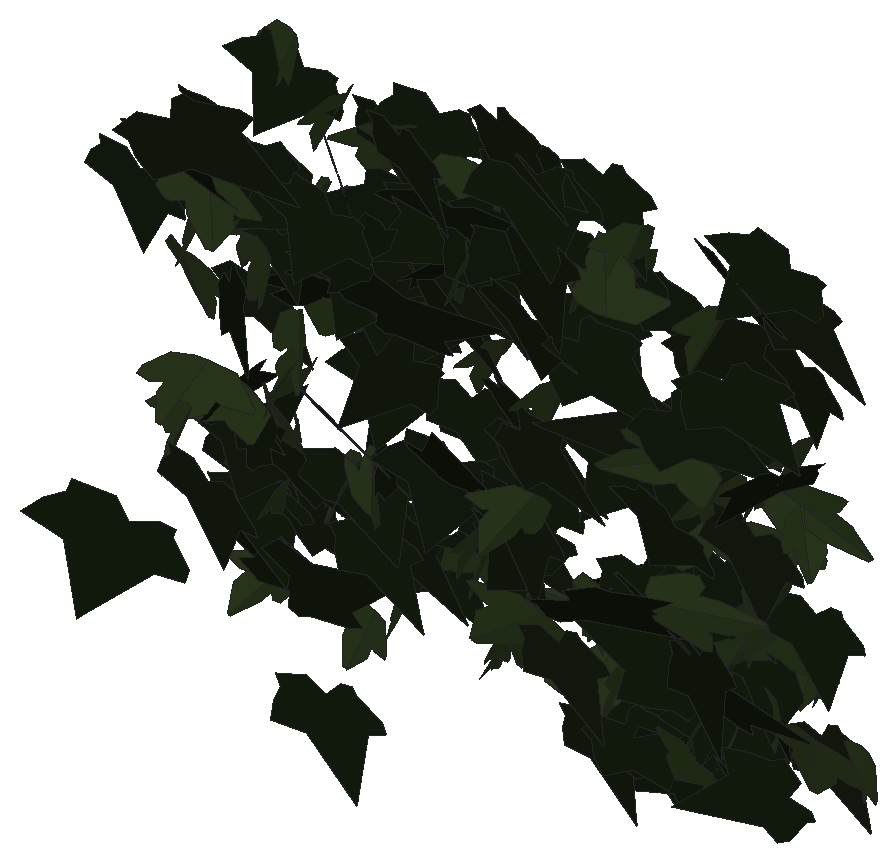
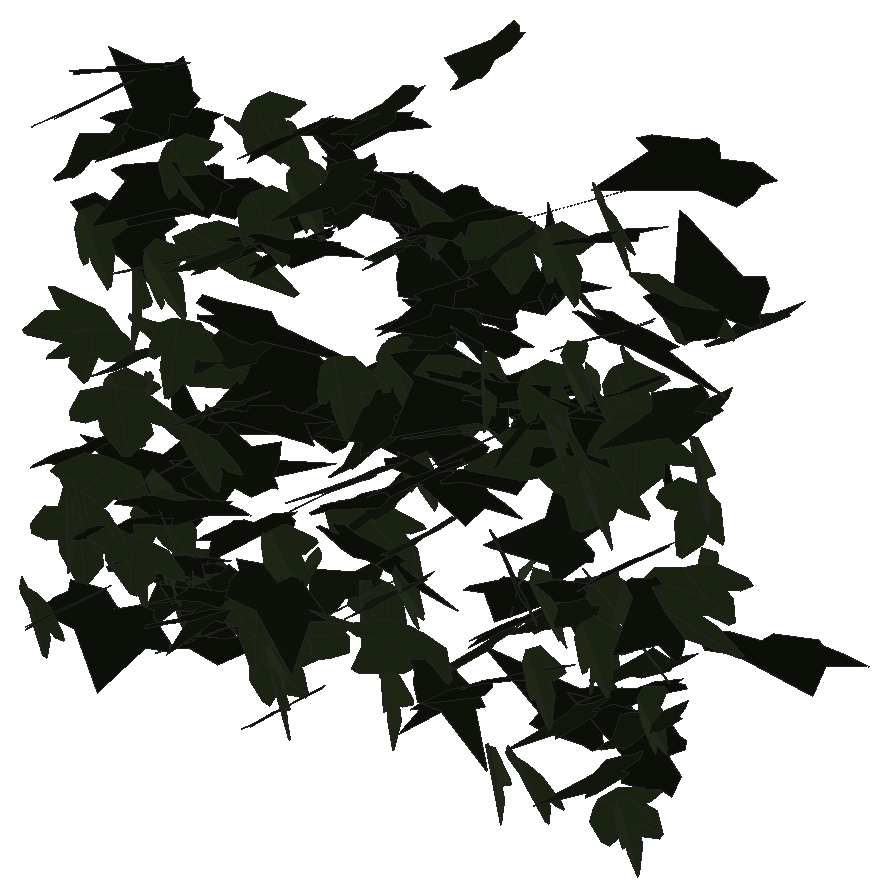
# SketchUp Ruby script. Lengths in millimetres.
U = 1.mm
M = Sketchup.active_model
def pt(a) = Geom::Point3d.new(a.map { |v| v * U })
def face(e, loops, mat)
  f = e.add_face(loops[0].map { |a| pt(a) })
  loops[1..].each { |l| e.add_face(l.map { |a| pt(a) }).erase! }
  f.material = f.back_material = mat if mat
  f
end
# faces: each face lists its corners as indices into pts; further lists are holes
def faces(e, pts, list, mat = nil) = list.each { |f| face(e, (f[0].is_a?(Array) ? f : [f]).map { |l| l.map { |i| pts[i] } }, mat) }
# xy, xz, yz: faces in a plane at the given z, y or x. An outline is a flat list of corners, or four numbers for a rectangle; further outlines are holes
def ring(l) = l.size == 4 ? [[l[0], l[1]], [l[2], l[1]], [l[2], l[3]], [l[0], l[3]]] : l.each_slice(2).to_a
def flat(e, list, mat, &to3) = list.each { |f| face(e, (f[0].is_a?(Array) ? f : [f]).map { |l| ring(l).map { |u, v| to3.(u, v) } }, mat) }
def xy(e, z, list, mat = nil) = flat(e, list, mat) { |x, y| [x, y, z] }
def xz(e, y, list, mat = nil) = flat(e, list, mat) { |x, z| [x, y, z] }
def yz(e, x, list, mat = nil) = flat(e, list, mat) { |y, z| [x, y, z] }
def lines(e, pts, list) = list.each { |a, b| e.add_line(pt(pts[a]), pt(pts[b])) }
# prism: a flat outline (further loops are holes) pulled along v
def prism(e, loops, v, mat = nil)
  f = face(e, loops, mat); d = Geom::Vector3d.new(v.map { |x| x * U })
  f.pushpull(f.normal.samedirection?(d) ? d.length : -d.length)
end
def box(e, o, s, mat = nil) = prism(e, [[o, [o[0] + s[0], o[1], o[2]], [o[0] + s[0], o[1] + s[1], o[2]], [o[0], o[1] + s[1], o[2]]]], [0, 0, s[2]], mat)
def at(x, y, z, deg = 0) = Geom::Transformation.translation(pt([x, y, z])) * Geom::Transformation.rotation(ORIGIN, Z_AXIS, deg.degrees)
def axes(o, x, y, z) = Geom::Transformation.new([*x, 0, *y, 0, *z, 0, *pt(o).to_a, 1])
def part(name) = M.definitions.add(name)
# library, detail: a bought-in or finely detailed component or shape, given as its bounding box
def library(name, o, s) = part(name).tap { |d| box(d.entities, o, s) }
def detail(e, o, s) = box(e.add_group.entities, o, s)
def put(e, d, t, mat = nil) = e.add_instance(d, t).tap { |i| i.material = mat if mat }
def group(e, t, mat = nil) = e.add_group.tap { |g| g.transformation = t; g.material = mat if mat }.entities
root = M.entities
M.materials.add("efeu1").color = [18, 25, 13]
M.materials.add("efeu2").color = [43, 57, 29]
c1 = part("ivyleaf_9")
p = [[39.1,54.8,31.7],[34.5,51.8,30.2],[-5.3,25.2,17.3],[-17.9,28.3,20.9],[-21.6,21.7,17],[-20.2,4.3,5.3],
  [-22.9,-0.3,2.5],[-17.1,-4,-0.6],[-2,-2.1,-1.2],[-0.7,-15.4,-10.1],[16.6,-22.3,-16.7],[21.1,-15.1,-12.5],
  [32.7,-10.7,-11],[46.1,-1.8,-6.6],[30.8,11.2,3.8]]
faces(c1.entities,p,[[0,1,2,3,4,5,6,7,8,9,10,11,12,13,14]],"efeu1")
c2 = part("ivyleaf_10")
p = [[0,12.8,-0.8],[-1.5,51.3,-10.9],[-4.9,51,-11.6],[-13.6,26.5,-7.3],[-13.2,15.9,-4.6],[-21.1,19.3,-7.2],
  [-29.5,16.3,-8.3],[-29.2,8.3,-6.2],[-19.7,-9.8,0.5],[-7.6,-13,4],[1,-12.2,5.8],[-0.4,51.1,-11.1],
  [-1.5,51.1,-10.9],[1,-12.4,5.9],[16.9,-12.4,3.5],[35.1,9.1,-5.1],[35,12.9,-6.1],[20.5,16.4,-4.9],
  [15.8,15,-3.8],[15.3,27.6,-7.1],[12.8,31.3,-7.8]]
faces(c2.entities,p,[[0,1,2,3,4,5,6,7,8,9,10],[11,12,0,13,14,15,16,17,18,19,20]],"efeu2")
put(root,c1,axes([3604.9,738.4,3982.3],[1.88272,-0.57074,-0.41456],[-0.29368,0.52166,-1.0864],[1.31002,0.93719,0.35225]))
put(root,c2,axes([3637.7,685.4,3837.3],[-1.88787,0.74992,0.06036],[-0.10016,0.03047,-1.24349],[-1.42836,-0.99331,0.00742]))
put(root,c2,axes([3644.9,677.5,3890.1],[0.51277,-1.02488,-0.67232],[-0.23166,0.66259,-1.05883],[2.32126,0.29252,0.04284]))
put(root,c2,axes([3652.5,789.4,3503.2],[0.23719,-1.12383,-0.13995],[0.00297,0.14097,-1.1306],[2.1554,0.12348,0.01696]))
put(root,c1,axes([3663.2,542.2,3598.3],[-2.10736,-0.93895,-0.17797],[0.24512,0.12329,-1.45175],[1.80224,-1.11468,-0.01065]))
put(root,c2,axes([3691.6,684.1,3698.1],[1.43146,0.01163,-0.98265],[-1.86965,-0.02391,-0.7522],[-0.04958,1.23723,-0.0053]))
put(root,c2,axes([3667.6,658.6,3727.4],[1.82984,0.62706,-0.49269],[-0.78388,-0.27039,-1.14786],[-1.29964,1.04596,-0.00136]))
put(root,c2,axes([3661.5,740.5,3604.9],[0.52982,-1.05246,0.46755],[0.36618,-0.43175,-1.08643],[2.16098,0.3312,0.06946]))
put(root,c1,axes([3650.6,581.4,3995.7],[-0.35738,-1.13105,0.46989],[0.12022,-0.48369,-1.13902],[2.32788,-0.14866,0.13096]))
put(root,c2,axes([3680.3,735.8,3921.3],[-1.6664,-0.81148,-0.09942],[0.10252,0.0881,-1.19346],[1.55257,-0.87679,-0.0279]))
put(root,c1,axes([3657.5,751.3,3585.3],[-0.0805,-1.07311,0.48491],[0.30202,-0.48599,-1.06166],[2.22073,0.02719,0.16196]))
put(root,c1,axes([3686.2,685.1,3698.8],[-0.4336,0.41966,-1.141],[-1.00594,1.01122,0.47746],[2.08366,0.57552,-0.00693]))
put(root,c1,axes([3659.4,756.8,3796.1],[0.55357,-1.07246,-0.43117],[-0.04514,0.43898,-1.10789],[2.19943,0.27894,0.08578]))
put(root,c2,axes([3684.2,608.3,3701.3],[0.95791,-1.06163,0.34009],[0.30189,-0.30114,-1.17482],[2.10005,0.52754,0.01376]))
put(root,c2,axes([3705.2,740.6,3472.7],[-0.68014,-0.69954,0.92647],[-0.06559,-0.96255,-0.74008],[2.20846,-0.24402,0.26334]))
put(root,c1,axes([3674.1,773.6,3542.6],[1.32044,-0.80727,-0.48232],[-0.18349,0.53516,-1.0344],[1.78031,0.6539,0.25112]))
put(root,c1,axes([3694.9,722.9,3629.2],[-0.90107,-0.9157,0.59609],[0.18785,-0.68283,-0.97056],[2.07098,-0.33648,0.34739]))
put(root,c2,axes([3710.5,775.6,3689.7],[-0.00606,-1.1655,0.03473],[0.00107,-0.03473,-1.16551],[2.21917,-0.00317,0.00066]))
put(root,c1,axes([3662.8,711.8,3541],[1.26369,-0.12698,-1.09291],[2.09388,0.06232,0.66117],[-0.02347,-1.27728,0.14091]))
put(root,c2,axes([3711.8,725.9,3917.1],[-0.02312,-1.12219,0.41483],[0.31578,-0.41243,-1.11082],[2.25501,0.04625,0.15981]))
put(root,c1,axes([3676.7,596.5,4012],[2.38837,-0.45203,-0.48301],[0.86203,-0.16782,1.33385],[-0.91765,-1.33416,-0.00413]))
put(root,c1,axes([3709.1,690.9,3643.6],[-0.70552,1.0118,0.57922],[0.33296,-0.55264,1.07734],[2.19376,0.40928,0.02277]))
put(root,c2,axes([3727.5,753.2,3850.9],[0.73278,-1.13199,0.04812],[0.01342,-0.04843,-1.19564],[2.15631,0.38499,-0.00891]))
put(root,c2,axes([3728.3,743.5,3860.6],[-2.27564,0.01771,-0.08918],[0.16884,-0.03049,-1.19547],[-0.03792,-1.19863,0.02909]))
put(root,c1,axes([3718,690.9,3588.5],[-0.28536,-1.13905,-0.28751],[0.16813,0.27809,-1.1478],[2.22951,-0.16676,0.04976]))
put(root,c2,axes([3738.9,726.7,3665],[0.63551,-0.86688,-0.74676],[0.0709,0.78574,-0.89547],[2.17644,0.22753,0.24722]))
put(root,c2,axes([3743.6,693,3695.5],[-1.46377,0.90288,0.31585],[-0.39084,0.23998,-1.18605],[-1.77802,-0.79605,0.00069]))
put(root,c2,axes([3747.4,671.9,3937],[-0.2984,-1.22936,0.23126],[0.02178,-0.23447,-1.23866],[2.38065,-0.15194,0.04032]))
put(root,c1,axes([3778.5,659.1,3991.4],[-2.3344,0.13213,0.29706],[-0.5601,0.04156,-1.23362],[-0.26298,-1.26134,-0.00953]))
put(root,c2,axes([3748,718.2,3950],[1.17324,-1.04031,0.07335],[0.0587,-0.06699,-1.20922],[1.98397,0.61718,-0.0076]))
put(root,c2,axes([3733.1,588.9,4004.2],[2.28453,-0.19085,0.29262],[0.5515,-0.04099,-1.21543],[0.37139,1.23483,0.00488]))
put(root,c1,axes([3725,640,3858],[-0.3236,-0.1695,-1.27422],[2.254,-0.52035,-0.08882],[-0.9511,-1.17549,0.22305]))
put(root,c1,axes([3738.6,689.5,3937.3],[-0.05824,-1.24024,-0.05442],[0.00692,0.05435,-1.24062],[2.36269,-0.03073,0.00229]))
put(root,c2,axes([3763.8,680.6,4141.4],[1.40023,-1.02372,0.03362],[0.05153,-0.02195,-1.26064],[1.94872,0.73617,0.00918]))
put(root,c2,axes([3769.9,671,3628.4],[0.16317,-1.08727,-0.50464],[0.04227,0.50728,-1.08919],[2.28093,0.06838,0.05628]))
put(root,c1,axes([3774.4,692.9,4112.1],[-1.26924,-0.9572,0.41119],[-0.16554,-0.43536,-1.15454],[1.9758,-0.65137,0.16742]))
put(root,c1,axes([3749.3,729.6,3568.5],[1.28842,-0.82498,-0.51444],[-0.2594,0.54014,-1.04556],[1.83209,0.65665,0.21374]))
put(root,c2,axes([3777.6,725.9,3891.6],[1.27672,-1.02597,0.04185],[0.02823,-0.0403,-1.22578],[1.95405,0.67092,-0.00964]))
put(root,c2,axes([3785.4,614.5,3918.7],[1.10417,-1.01804,-0.39809],[-0.09694,0.42503,-1.16114],[2.07815,0.56074,0.15736]))
put(root,c1,axes([3793.1,681,3975.6],[-1.30089,-0.64737,0.81932],[-0.54729,-0.82468,-0.89151],[1.9105,-0.67705,0.3025]))
put(root,c2,axes([3785.3,711.3,3959.5],[0.72876,-1.08925,0.4376],[0.32325,-0.40404,-1.15433],[2.21059,0.41817,0.02453]))
put(root,c2,axes([3793.2,730.7,3883.1],[0.71843,-1.14486,-0.10282],[-0.00767,0.1069,-1.20513],[2.18766,0.37635,0.02954]))
put(root,c2,axes([3802.4,752.2,3613.1],[0.15499,-1.17825,-0.16844],[-0.03551,0.16755,-1.18104],[2.26497,0.08325,-0.00699]))
put(root,c1,axes([3760.2,504.6,4125.5],[0.16109,-0.49814,-1.31185],[0.92699,1.24295,-0.44055],[2.50461,-0.42799,0.24743]))
put(root,c2,axes([3806.3,742.6,3946.7],[-0.31929,-1.10569,0.46803],[0.11828,-0.47994,-1.11155],[2.28205,-0.12982,0.12309]))
put(root,c1,axes([3783.4,666.8,3661.8],[1.66208,-0.76684,-0.3514],[-0.17777,0.41478,-1.13728],[1.59551,0.84504,0.23935]))
put(root,c2,axes([3819.8,696.2,4086.9],[-0.03401,-1.23895,0.12133],[0.01779,-0.12147,-1.23903],[2.36919,-0.01687,0.01104]))
put(root,c1,axes([3776.7,678.1,3858.4],[1.53277,0.85603,-0.56737],[0.75341,0.40655,1.1753],[1.80352,-0.89736,-0.00877]))
put(root,c2,axes([3801.1,649.5,3835],[1.23526,-0.79377,0.75091],[1.08248,-0.50031,-1.02049],[1.77563,0.85721,0.09973]))
put(root,c1,axes([3863.9,745.1,3913.7],[-1.63684,-0.17057,0.82517],[-1.49382,-0.26669,-0.8732],[0.58329,-1.16166,0.07931]))
put(root,c1,axes([3786.8,667.2,3508.9],[-0.15083,0.05703,1.23905],[2.17279,-0.48202,0.09521],[0.92287,1.14419,-0.02165]))
put(root,c2,axes([3832.7,596.7,3816.9],[0.65226,-1.17563,0.02611],[0.00782,-0.026,-1.22456],[2.238,0.34273,-0.00333]))
put(root,c2,axes([3836.2,723.7,3465.1],[1.67791,-0.72881,0.01205],[0.00951,-0.01287,-1.14385],[1.38724,0.88161,-0.00673]))
put(root,c2,axes([3839.9,694.5,3659.9],[0.91357,-1.0968,0.32795],[0.18642,-0.31496,-1.19672],[2.17075,0.48864,-0.03524]))
put(root,c1,axes([3802.7,678.6,3733.8],[1.75457,-0.84276,0.21842],[0.29752,-0.1527,-1.24904],[1.63,0.93504,-0.00712]))
put(root,c1,axes([3836.4,754.3,3590.6],[-0.86889,-1.04318,0.27442],[0.05312,-0.30932,-1.12939],[2.05225,-0.43366,0.14542]))
put(root,c1,axes([3841.9,698.3,3900.5],[1.31419,-0.30849,-0.95222],[-1.39455,0.63231,-0.7362],[1.29779,0.99183,0.17317]))
put(root,c2,axes([3820.5,705.4,3841.3],[-1.13649,-0.30203,-1.00849],[1.77482,0.38625,-0.66786],[0.92972,-1.10655,0.04215]))
put(root,c2,axes([3859.5,750,3479.2],[0.39591,-0.92707,-0.71091],[-0.23831,0.70024,-0.9498],[2.21065,0.24152,0.02493]))
put(root,c1,axes([3856.1,704.4,3891.7],[-0.96978,-0.97476,0.52143],[-0.07156,-0.55854,-1.08088],[2.1027,-0.46858,0.2037]))
put(root,c1,axes([3843.4,670.5,4016.4],[-0.07899,-0.17225,1.30547],[-0.09997,-1.30486,-0.17384],[2.50411,-0.05753,0.03424]))
put(root,c2,axes([3870.2,745.9,3943.6],[0.20665,-1.02035,-0.63494],[0.07123,0.64009,-1.02222],[2.28611,0.07229,0.08924]))
put(root,c1,axes([3848.3,449.2,3751.7],[-0.15399,-1.18047,0.66258],[0.21565,-0.66733,-1.17511],[2.56732,-0.01475,0.13845]))
put(root,c1,axes([3886.4,681.3,3659.4],[0.19705,0.28094,1.16639],[-0.05465,1.17097,-0.27949],[-2.2827,-0.00378,0.10738]))
put(root,c1,axes([3854.4,691.1,3665.5],[-0.66281,-1.04427,-0.57352],[0.51294,0.51298,-1.09769],[2.20869,-0.43251,0.08282]))
put(root,c2,axes([3889.6,660.1,3653.1],[0.29183,0.52626,-1.12057],[-0.21195,1.13041,0.51564],[2.34659,0.03665,0.18593]))
put(root,c1,axes([3875.9,702.8,3911.9],[-1.27257,-0.97782,-0.33325],[0.28678,0.3004,-1.18378],[1.94507,-0.68403,-0.0435]))
put(root,c2,axes([3894,694.3,4075.4],[-1.30509,-0.99875,0.1184],[-0.06987,-0.11835,-1.21095],[1.91285,-0.68574,0.03655]))
put(root,c1,axes([3909.8,734.2,3911],[-2.08795,-0.48625,0.11292],[-0.22557,-0.01113,-1.19941],[0.92289,-1.10282,-0.03768]))
put(root,c1,axes([3872.3,719,4069.4],[0.36762,-1.19003,0.23852],[0.06267,-0.23629,-1.20559],[2.30906,0.19587,-0.00525]))
put(root,c1,axes([3923.4,685.5,3998.6],[-0.5963,-0.64155,-1.03911],[-0.23663,-1.05043,0.68603],[-2.31211,0.27296,0.19778]))
put(root,c2,axes([3913.5,730.1,3913.3],[-2.26178,0.01105,0.20206],[-0.38511,-0.0512,-1.18731],[-0.00437,-1.20438,0.05232]))
put(root,c1,axes([3900.5,704.8,3793.7],[-1.13836,-1.04604,0.07859],[-0.05532,-0.0739,-1.20492],[1.99567,-0.59872,0.01143]))
put(root,c1,axes([3889.6,735.8,3842.8],[-0.05022,-1.19226,0.13828],[0.0338,-0.13868,-1.19238],[2.28408,-0.02416,0.02069]))
put(root,c1,axes([3887.4,669.4,3605.1],[0.35691,-1.14588,-0.32734],[0.00758,0.33197,-1.15981],[2.26808,0.17921,0.05539]))
put(root,c1,axes([3930.7,745.7,3550.7],[-0.50517,1.1221,-0.04837],[0.03456,-0.04541,-1.15305],[-2.13729,-0.26595,-0.00721]))
put(root,c1,axes([3891.9,714,3591.4],[0.88606,-1.0279,-0.3823],[-0.15822,0.38105,-1.12578],[2.08122,0.46659,0.07718]))
put(root,c1,axes([3896.8,759.1,3553.7],[0.42245,-0.98217,-0.60833],[-0.12359,0.60787,-1.00512],[2.19529,0.22322,0.06048]))
put(root,c1,axes([3913.3,759.6,3857.2],[-1.13155,-0.94767,0.40441],[0.11837,-0.49907,-1.07804],[1.95739,-0.51766,0.29898]))
put(root,c1,axes([3914.3,566.9,4041.8],[-1.00586,-1.00941,0.55527],[-0.13483,-0.58128,-1.12412],[2.18844,-0.49976,0.18595]))
put(root,c1,axes([3938.4,668.8,3831.4],[-2.35089,0.22734,-0.40711],[0.75934,-0.08129,-1.25595],[-0.45929,-1.29805,0.00736]))
put(root,c1,axes([3957.7,574.1,4003.4],[-1.23802,1.03551,0.3217],[-0.37542,0.25588,-1.22251],[-2.02927,-0.67909,0.0299]))
put(root,c1,axes([3907.6,725.6,3903.4],[2.19798,0.34027,0.01562],[-0.02313,0.09635,-1.20015],[-0.64786,1.15097,0.09585]))
put(root,c1,axes([3927.6,729.5,4092.9],[-0.74225,-1.1564,0.05245],[-0.04128,-0.04804,-1.22038],[2.20274,-0.39057,-0.0052]))
put(root,c1,axes([3937.3,773,3729.1],[0.37026,-1.15045,-0.03245],[-0.00602,0.03238,-1.16678],[2.1904,0.19456,0.00228]))
put(root,c1,axes([3944.9,692.8,3990.3],[0.65759,-0.66975,-0.96332],[-0.20179,0.98229,-0.72097],[2.22381,0.28718,0.21944]))
put(root,c1,axes([3932.3,689.4,3949.4],[-0.02407,-0.70865,-1.00065],[1.4773,0.77004,-0.55514],[1.80651,-0.63915,0.44064]))
put(root,c1,axes([3966.5,496.5,3517.8],[-0.18034,-1.31976,-0.20399],[0.04395,0.20285,-1.32313],[2.54122,-0.09716,0.00841]))
put(root,c1,axes([4004.7,659.4,3982.2],[-0.15646,1.21274,-0.3604],[0.03356,-0.36002,-1.21551],[-2.40761,-0.08383,0.00648]))
put(root,c2,axes([3974.4,749.1,3582.4],[-1.78879,-0.3132,-0.59798],[1.18517,-0.00665,-0.97531],[0.49587,-1.11396,0.17395]))
put(root,c1,axes([4010.6,659.7,4021.1],[-1.5739,-0.61661,0.73916],[-0.83913,-0.6236,-1.0135],[1.62851,-0.91726,0.19214]))
put(root,c1,axes([3975.1,728.5,3771.1],[-0.04254,-1.20348,-0.10073],[0.04284,0.10032,-1.20351],[2.29808,-0.02415,0.02057]))
put(root,c1,axes([3964.8,684.9,3926],[0.9929,-1.14333,0.15498],[0.11762,-0.14215,-1.25673],[2.19274,0.52534,-0.00276]))
put(root,c1,axes([4013.6,641.8,4051.9],[1.36291,0.6531,-0.8491],[-1.2425,-0.54368,-0.96878],[-1.61639,0.96861,0.02874]))
put(root,c1,axes([4002.2,662.6,3733.8],[-2.02477,-0.42242,-0.52722],[0.9753,0.13628,-1.14326],[0.83782,-1.1795,0.05673]))
put(root,c1,axes([3958.2,600.3,3926.9],[0.29881,-0.2934,1.28344],[2.21806,-0.57029,-0.27293],[1.16557,1.16045,0.19036]))
put(root,c2,axes([3999.1,686.3,4066.1],[1.98127,-0.56831,0.28773],[0.45713,-0.16037,-1.18579],[1.12285,1.06808,-0.02495]))
put(root,c2,axes([4018.1,725.6,3505.1],[0.2314,-1.0763,-0.59242],[-0.06481,0.59213,-1.08277],[2.33732,0.12297,0.02863]))
put(root,c2,axes([4007.1,716,3624.7],[0.75249,-0.93989,0.65121],[0.50004,-0.59593,-1.01963],[2.11798,0.47463,0.00936]))
put(root,c1,axes([4000.8,747.3,3624.6],[-0.04401,-1.1499,0.25377],[0.04766,-0.25424,-1.14975],[2.24064,-0.01718,0.02944]))
put(root,c2,axes([4035.7,692.2,3874.6],[-0.24942,-1.21928,0.03461],[-0.0059,-0.03448,-1.22631],[2.32147,-0.13109,0.0006]))
put(root,c2,axes([4034.4,710.9,3533.3],[0.22484,-1.09145,-0.44038],[0.16118,0.44932,-1.09091],[2.23415,0.07742,0.12302]))
put(root,c2,axes([4038,632.1,3999.4],[0.52189,-1.14773,-0.41918],[0.15198,0.44552,-1.16761],[2.32051,0.22895,0.17074]))
put(root,c1,axes([4078.3,721.5,3657],[-2.12201,0.25235,0.30009],[-0.55615,0.06832,-1.14317],[-0.49755,-1.15263,-0.00206]))
put(root,c1,axes([4018.4,743.8,3626.9],[0.95126,-0.86949,-0.61124],[-0.20464,0.63063,-0.98499],[2.01242,0.47513,0.18877]))
put(root,c1,axes([4044.1,629.3,3737.5],[1.86003,-0.73267,0.40156],[-0.5847,0.25954,1.22125],[-1.47871,-1.02423,0.02221]))
put(root,c1,axes([4020.6,551.4,4176.4],[0.67205,-1.18551,0.29194],[0.07646,-0.29246,-1.2362],[2.32241,0.35269,-0.04378]))
put(root,c2,axes([4067.3,674,3567],[-1.76791,0.77239,0.36964],[-0.5269,0.24518,-1.20803],[-1.54215,-0.96923,-0.01101]))
put(root,c1,axes([4032.6,707.4,3811.1],[1.39009,-0.95556,-0.00697],[-0.0226,-0.0003,-1.20269],[1.81852,0.73043,-0.00962]))
put(root,c1,axes([4037.8,661,4001],[0.48636,-1.32619,-0.01949],[-0.00844,0.019,-1.35059],[2.52427,0.25559,-0.00076]))
put(root,c1,axes([4034.4,736.2,3754.1],[0.94191,-0.96743,-0.49733],[0.10908,0.56881,-1.04946],[2.06738,0.41076,0.28196]))
put(root,c2,axes([4065.6,707.3,3584.2],[0.39401,-1.06992,-0.47692],[0.15482,0.49627,-1.07802],[2.22403,0.155,0.15953]))
put(root,c1,axes([4068.2,722.2,3707.7],[-0.89236,-1.07306,0.3067],[-0.14375,-0.3014,-1.16997],[2.11917,-0.4723,0.04979]))
put(root,c2,axes([4083,608.9,3709.8],[0.23523,-1.20506,0.1788],[-0.00623,-0.18005,-1.21119],[2.31856,0.12178,-0.02139]))
put(root,c1,axes([4056.6,672.3,4152.9],[0.9838,-1.14167,-0.11825],[-0.03167,0.12223,-1.25275],[2.18423,0.51599,0.0351]))
put(root,c1,axes([4106.8,658.8,4053.8],[-2.27874,-0.19335,-0.15528],[0.29767,0.00537,-1.21267],[0.36625,-1.20733,0.01947]))
put(root,c1,axes([4062.5,722.5,4091.1],[1.68977,-0.7157,-0.48462],[-0.36136,0.51628,-1.11031],[1.60483,0.86983,0.26026]))
put(root,c1,axes([4084.6,669.4,3658.8],[-0.59551,-0.66714,1.03647],[-0.35291,-1.0317,-0.72004],[2.31922,-0.32829,0.15657]))
put(root,c2,axes([4096.8,709.9,3841.2],[-0.42635,-1.19245,-0.19776],[0.07174,0.19414,-1.21331],[2.29935,-0.22717,0.00118]))
put(root,c2,axes([4136.3,620.9,3618.9],[-1.78537,-0.08041,0.78306],[-1.42146,-0.29386,-0.92492],[0.47322,-1.1861,0.17606]))
put(root,c2,axes([4149,770.3,3554.8],[0.40202,0.29077,1.11553],[-1.55349,-0.76313,0.35348],[1.54931,-0.84063,0.06497]))
put(root,c1,axes([4131.3,770,3602.3],[0.29224,1.16271,-0.02225],[0.03495,-0.02487,-1.17261],[-2.21301,0.15315,-0.02146]))
put(root,c1,axes([4101.4,647.4,3722.5],[0.07501,-1.2902,0.50679],[-0.04696,-0.50757,-1.29026],[2.63773,0.02765,-0.03738]))
put(root,c1,axes([4107.6,783.5,3473.8],[0.24871,-1.1403,-0.10433],[-0.04047,0.10258,-1.14773],[2.17891,0.13207,-0.00941]))
put(root,c1,axes([4114.9,659,4115.3],[-0.81434,-1.25234,-0.27887],[0.24344,0.25086,-1.32284],[2.42967,-0.44487,0.03907]))
put(root,c1,axes([4107.2,648.5,3813.6],[1.17801,-0.95162,-0.6698],[-0.4278,0.64659,-1.12638],[2.17306,0.64317,0.14135]))
put(root,c2,axes([4141.9,600.5,3764.2],[-0.83327,-0.87738,0.74683],[-0.08169,-0.78596,-0.94851],[2.19133,-0.36293,0.24863]))
put(root,c1,axes([4107.8,690.2,3561.9],[0.11342,-1.11553,0.60498],[0.38854,-0.58933,-1.10679],[2.38375,0.14914,0.15162]))
put(root,c2,axes([4131,716.1,3601.1],[-0.45938,1.13588,-0.00602],[0.01258,-0.00475,-1.16123],[-2.16181,-0.2414,-0.00548]))
put(root,c2,axes([4145.9,753.9,3480.8],[0.83341,-1.02538,-0.32714],[-0.06254,0.34027,-1.11054],[2.04745,0.42777,0.09924]))
put(root,c1,axes([4121.4,639.9,4043.3],[-1.23104,-0.14753,-1.1372],[2.17564,0.0202,-0.65283],[0.17243,-1.30813,0.11817]))
put(root,c2,axes([4132.8,712.2,3496.7],[1.29366,0.71896,-0.67941],[0.90478,0.48548,0.98936],[1.65096,-0.82942,-0.00983]))
put(root,c1,axes([4143,738.8,3997.5],[-1.30319,-0.95309,-0.27578],[0.59048,0.1126,-1.15947],[1.79365,-0.72955,0.18133]))
put(root,c2,axes([4160.3,752,3489.9],[-0.17298,-0.84923,0.82594],[0.06618,-0.82992,-0.8495],[2.25363,-0.04081,0.08834]))
put(root,c2,axes([4172.3,767.8,3553.4],[-1.59821,0.78211,0.26976],[-0.66229,0.01481,-1.1262],[-1.42851,-0.88189,0.22033]))
put(root,c2,axes([4169,719.8,3613.7],[-0.06716,-1.1537,0.20714],[-0.03639,-0.20664,-1.15417],[2.23053,-0.03811,-0.01259]))
put(root,c2,axes([4158.3,743.5,3508.1],[0.57932,-0.91835,0.667],[0.50344,-0.61416,-0.96631],[2.10068,0.40045,0.04764]))
put(root,c1,axes([4144.5,611.9,3978.4],[-0.40297,-0.90489,0.90272],[0.4391,-0.92705,-0.87516],[2.39266,0.01773,0.31264]))
put(root,c2,axes([4173.4,683.1,4025.1],[0.51175,-1.18359,0.29569],[0.09542,-0.29181,-1.21366],[2.31988,0.2731,-0.01531]))
put(root,c2,axes([4184.4,716.5,3604],[0.28044,-1.16182,-0.19247],[0.06573,0.19815,-1.16967],[2.24035,0.13962,0.05841]))
put(root,c1,axes([4192.4,739.8,3775],[-1.74073,-0.73767,0.16139],[-0.1736,-0.14371,-1.17379],[1.42662,-0.91758,0.05409]))
put(root,c1,axes([4160.9,713.3,4106.8],[0.20556,-1.22719,-0.215],[-0.01857,0.21496,-1.23191],[2.3711,0.10807,0.00899]))
put(root,c2,axes([4188.8,726.1,4014.5],[-0.51771,-1.16742,0.29223],[-0.00004,-0.2996,-1.19687],[2.29039,-0.26389,0.06603]))
put(root,c1,axes([4170.8,693,3962.7],[0.25898,-1.1957,-0.33329],[-0.09665,0.32964,-1.20335],[2.36043,0.14469,-0.01271]))
put(root,c1,axes([4206.2,765.7,3566.4],[-1.43473,-0.89375,-0.0152],[0.10232,-0.02549,-1.16781],[1.69815,-0.75358,0.05753]))
put(root,c1,axes([4183.4,675.4,3479.5],[0.34755,-1.20725,0.10411],[0.03506,-0.10251,-1.22098],[2.3059,0.18352,0.00287]))
put(root,c1,axes([4191.9,737.9,3641.5],[-0.00174,-1.05831,-0.50356],[-0.00509,0.50356,-1.05831],[2.23055,0.00032,-0.00281]))
put(root,c1,axes([4196.8,595.2,3618.1],[0.29931,-1.22297,-0.12797],[0.01217,0.12983,-1.23283],[2.34022,0.15574,0.02278]))
put(root,c1,axes([4268.6,689.5,3840.8],[-1.69257,0.12566,0.81012],[-1.54367,0.03894,-0.89644],[-0.22689,-1.20237,0.05563]))
put(root,c2,axes([4228.2,635.6,4022.7],[2.32562,-0.11879,0.25277],[-0.44925,0.16708,1.21964],[-0.2841,-1.23659,0.14051]))
put(root,c1,axes([4203.9,623.6,3964.3],[0.61573,-0.9443,-1.00575],[-0.22205,1.01061,-0.98639],[2.61621,0.30801,0.15299]))
put(root,c1,axes([4199.3,751,3970.7],[0.87877,-1.07055,-0.28617],[0.14708,0.34037,-1.14863],[2.10388,0.42337,0.19983]))
put(root,c2,axes([4235.2,668.2,4084.6],[-0.35922,-1.12984,0.47136],[0.26675,-0.49374,-1.12735],[2.31461,-0.11844,0.20307]))
put(root,c1,axes([4232.1,729.7,3484.9],[-0.81973,-1.05196,-0.21086],[0.323,0.15756,-1.13268],[2.01621,-0.45294,0.09573]))
put(root,c1,axes([4236.8,753.8,3764.2],[-0.68319,-1.02949,0.48739],[0.00786,-0.51219,-1.07884],[2.16779,-0.32259,0.15751]))
put(root,c1,axes([4234.6,725.7,3541.9],[1.55332,-0.47565,-0.74425],[-1.0214,0.53778,-0.93222],[1.33513,0.96479,0.1527]))
put(root,c1,axes([4256.9,775.8,3522.4],[-1.12664,-0.84479,0.49042],[-0.26497,-0.49462,-1.02009],[1.84011,-0.58846,0.15337]))
put(root,c1,axes([4250.9,748.3,3490.1],[-0.45491,-1.11984,0.32087],[0.04779,-0.33243,-1.14148],[2.21652,-0.22267,0.09047]))
put(root,c2,axes([4263.6,746,3724.7],[2.03367,-0.54273,-0.06312],[-0.10658,0.02912,-1.19848],[1.03441,1.07002,0.00061]))
put(root,c1,axes([4243.1,651.1,3512],[0.30947,-0.85196,-0.84036],[0.0835,0.85176,-0.85502],[2.27599,0.08459,0.14563]))
put(root,c1,axes([4246.9,560.1,3703.7],[2.30361,0.63768,0.61607],[0.99599,0.32779,-1.36745],[-1.36223,1.31801,0.04201]))
put(root,c1,axes([4260.7,681.2,3640],[-0.44161,-0.6704,1.11977],[0.80363,-1.11472,-0.57988],[2.35029,0.25519,0.40868]))
put(root,c1,axes([4270.1,671.7,3461.3],[-0.44897,-0.15567,1.19531],[1.9243,0.63758,0.28258],[-1.24904,1.03822,0.00569]))
put(root,c1,axes([4276.2,756.3,3646],[-1.05386,-1.01419,-0.31515],[0.57414,0.19057,-1.14333],[1.938,-0.60796,0.16734]))
put(root,c1,axes([4334,635.8,3611.3],[-1.51632,-0.92263,-0.46111],[-0.5792,-0.34644,1.21901],[-1.87564,0.85286,-0.00366]))
put(root,c1,axes([4323.8,666.3,3489.5],[-1.63243,0.78078,-0.06225],[0.07571,-0.04876,-1.15984],[-1.48878,-0.8586,0.00927]))
put(root,c2,axes([4298.3,696.7,3515.1],[0.35658,-1.05396,-0.44715],[0.10558,0.46092,-1.06318],[2.17639,0.15032,0.12484]))
put(root,c1,axes([4295.9,658.8,3765.8],[-0.98204,-0.70657,0.92485],[0.19615,-1.03544,-0.73355],[2.20638,-0.22244,0.47686]))
put(root,c2,axes([4338.6,621.6,3876.7],[1.38182,0.11446,-1.00994],[-1.92911,-0.01047,-0.72987],[-0.14339,1.2438,0.0868]))
put(root,c2,axes([4334.4,646.1,3501.9],[-1.64445,0.37667,0.68619],[-1.25004,0.20714,-0.94075],[-0.81046,-1.08376,0.05869]))
put(root,c1,axes([4315.2,752.4,3559.4],[-1.47897,-0.87318,0.27668],[-0.15856,-0.29396,-1.16169],[1.73604,-0.77073,0.12961]))
put(root,c1,axes([4293.2,751.2,3677.1],[0.45973,-1.15797,-0.22132],[-0.07401,0.21797,-1.18288],[2.24252,0.24459,0.00633]))
put(root,c1,axes([4298.4,732.4,3501],[-0.36012,-0.91859,0.6675],[0.41243,-0.69348,-0.89292],[2.12138,-0.02111,0.28691]))
put(root,c2,axes([4330.1,723.2,3602.6],[-0.66657,-1.02209,0.44967],[-0.22678,-0.43437,-1.08012],[2.11304,-0.36904,0.02593]))
put(root,c1,axes([4330,737.1,3497.5],[-1.38659,-0.6525,0.6229],[-0.41816,-0.64821,-0.936],[1.66514,-0.70613,0.28364]))
put(root,c2,axes([4323.8,695.4,3801.1],[-0.65155,-1.11856,-0.45271],[0.33378,0.41946,-1.16902],[2.2722,-0.38236,0.04191]))
put(root,c2,axes([4331.8,703.5,3515.5],[0.7436,-1.01895,-0.39398],[-0.27236,0.36707,-1.09129],[2.06127,0.41609,-0.00207]))
put(root,c2,axes([4327.8,689.8,4010.7],[-0.25937,-1.16164,0.45441],[0.14734,-0.46411,-1.16321],[2.36938,-0.0983,0.12208]))
put(root,c2,axes([4335.6,717.1,3616.7],[0.74145,-1.14716,-0.05399],[-0.03351,0.05104,-1.21151],[2.18543,0.38998,-0.00026]))
put(root,c2,axes([4328.1,766.4,3580.3],[2.23047,-0.01511,0.0935],[0.18024,0.16889,-1.15972],[0.0028,1.16349,0.16955]))
put(root,c1,axes([4345.7,705,3527.3],[-1.45225,-0.8808,-0.0431],[0.05544,0.03178,-1.16536],[1.67742,-0.76361,0.00121]))
put(root,c1,axes([4340.4,707.1,3886.6],[-0.99656,-1.02596,0.45091],[0.05154,-0.50914,-1.12701],[2.13225,-0.4672,0.23799]))
put(root,c1,axes([4351.8,764.6,3492.2],[1.725,0.56279,-0.46541],[-1.01579,0.00415,-1.03439],[-0.94869,1.01887,0.26129]))
put(root,c1,axes([4327.2,691,3987],[-0.07752,-0.52572,-1.14109],[0.2701,1.13246,-0.52681],[2.37583,-0.1459,0.02266]))
put(root,c2,axes([4361.5,750.2,3732.4],[-1.86414,-0.65909,0.17702],[0.0271,-0.32933,-1.14737],[1.29854,-0.93929,0.27807]))
put(root,c2,axes([4366.2,725,3549.6],[1.30631,-0.78997,-0.53731],[-0.31909,0.55173,-1.02535],[1.79006,0.67483,0.20933]))
put(root,c2,axes([4364.4,681.2,3865.1],[0.3372,-1.18072,0.34133],[0.0415,-0.34179,-1.19362],[2.3388,0.1763,-0.02803]))
put(root,c1,axes([4356.4,756.7,3588.9],[-0.77917,-1.11067,0.00526],[-0.00174,-0.00527,-1.18373],[2.11386,-0.4094,0.00096]))
put(root,c1,axes([4342.6,604.8,3939.2],[0.35194,-0.51713,-1.20247],[0.09122,1.21627,-0.5157],[2.48953,0.02854,0.18889]))
put(root,c2,axes([4380.6,693.6,3839.1],[0.47753,-1.03158,-0.63435],[0.12131,0.65817,-1.04512],[2.30162,0.17934,0.1867]))
put(root,c1,axes([4343.7,689.8,4061.6],[0.44996,-0.65477,1.04571],[0.74763,-0.96938,-0.69579],[2.22595,0.45794,0.02231]))
put(root,c1,axes([4336.3,659.6,3588.3],[0.94035,-0.48091,1.03658],[1.47739,-0.68748,-0.68896],[1.59594,0.91977,0.02702]))
put(root,c1,axes([4371.5,699.5,3760.3],[-0.3351,-1.20745,0.37751],[0.10318,-0.388,-1.21571],[2.4055,-0.15156,0.10473]))
put(root,c2,axes([4345.3,597.4,3718.2],[0.49332,-0.06776,-1.21929],[2.29047,-0.19721,0.2668],[-0.39415,-1.23084,0.02437]))
put(root,c1,axes([4371.9,608,3657.4],[-1.04109,0.00334,-1.18883],[2.23066,-0.21759,-0.53992],[-0.37882,-1.29043,0.08796]))
put(root,c2,axes([4402.3,695.6,3708.8],[-0.15876,-1.17276,0.1863],[-0.03279,-0.18554,-1.17571],[2.25974,-0.08509,-0.00397]))
put(root,c1,axes([4411.8,700.5,4093.2],[-1.58942,-0.75422,0.51805],[-0.32715,-0.55958,-1.09178],[1.71042,-0.80789,0.27258]))
put(root,c2,axes([4393.6,759.9,3605.4],[1.80888,-0.68938,0.15691],[0.31385,-0.03949,-1.17237],[1.30846,0.9625,0.06429]))
put(root,c2,axes([4389.7,735.8,3632.9],[-1.42247,-0.70583,-0.57898],[1.01505,0.2697,-1.01727],[1.41012,-0.90615,0.14822]))
put(root,c2,axes([4399.3,655.7,3693.9],[0.6716,-0.86341,-0.86324],[0.40471,0.9283,-0.84156],[2.28815,0.08923,0.40222]))
put(root,c2,axes([4408.7,768.6,3593.6],[0.56966,-1.00342,-0.53711],[0.12773,0.56997,-1.0274],[2.16231,0.23068,0.20219]))
put(root,c1,axes([4395.7,782.9,3493.6],[0.37596,-1.11497,-0.23156],[-0.01808,0.2334,-1.13192],[2.16723,0.19537,0.03073]))
put(root,c2,axes([4415.6,728,3781.9],[0.47735,1.16247,-0.08142],[-0.20102,-0.06027,-1.18578],[-2.2087,0.25672,0.09032]))
put(root,c1,axes([4413,748,3660],[-0.28792,-1.19334,0.00205],[-0.04305,0.0008,-1.20268],[2.27076,-0.15129,-0.02254]))
put(root,c1,axes([4446.7,641.4,3885],[-0.24909,1.13232,-0.66665],[0.09997,-0.6649,-1.13966],[-2.49878,-0.13948,0.02086]))
put(root,c1,axes([4409,606.7,3997.1],[-0.07858,-0.87034,-0.91332],[0.26734,0.90496,-0.86872],[2.38615,-0.13005,0.06725]))
put(root,c2,axes([4436.3,702.1,3894.4],[0.00844,-1.23945,0.07256],[0.04558,-0.07247,-1.23923],[2.36252,0.00582,0.02365]))
put(root,c2,axes([4451.3,706.3,3534.2],[-2.13647,0.22492,0.28231],[-0.54466,0.00746,-1.14389],[-0.41866,-1.1575,0.04749]))
put(root,c2,axes([4399.6,730.6,3799.1],[1.2073,0.07075,1.00459],[1.79677,0.37156,-0.62231],[-0.66727,1.12852,0.14192]))
put(root,c2,axes([4443.5,785.7,3481.1],[1.49398,-0.84041,-0.06617],[0.14364,0.16011,-1.13821],[1.59798,0.77132,0.16417]))
put(root,c1,axes([4423.6,696,4055.5],[0.78072,-1.1087,-0.42821],[-0.00821,0.45161,-1.17341],[2.26197,0.38431,0.14354]))
put(root,c1,axes([4479.3,612.2,3530.7],[-1.51204,-0.34135,0.79792],[-1.21174,-0.50589,-0.85035],[1.12246,-1.00595,0.15688]))
put(root,c1,axes([4432.1,705.1,3980],[0.00516,-1.0552,0.65451],[0.052,-0.6543,-1.05497],[2.36263,0.01671,0.02179]))
